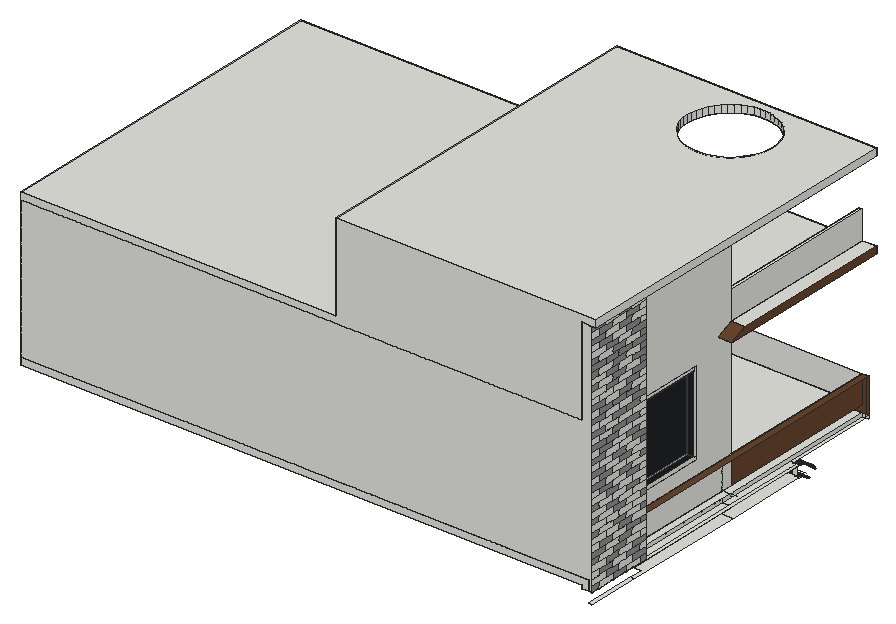
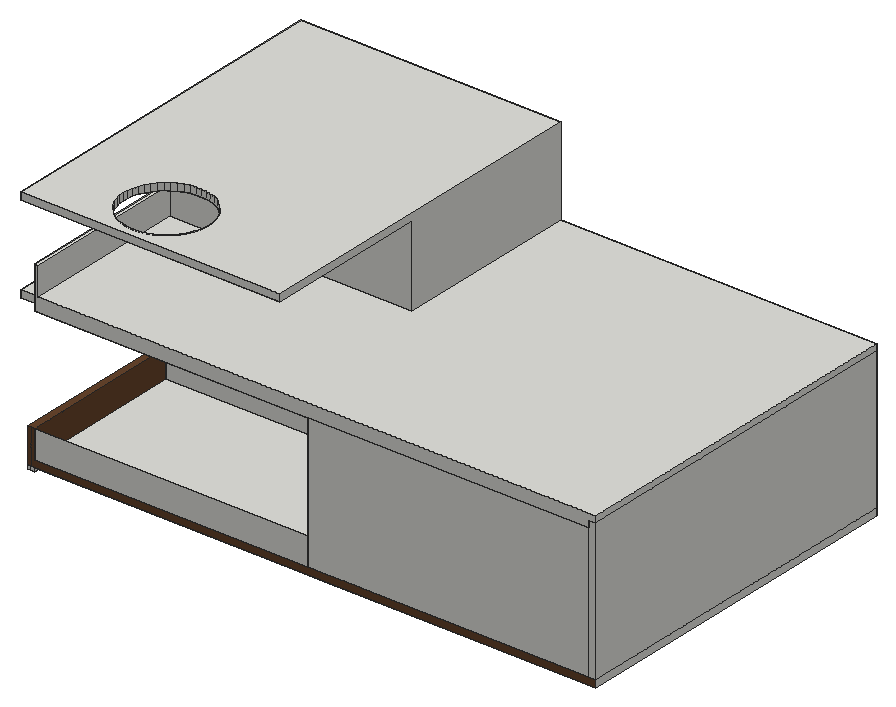
# SketchUp Ruby script. Lengths in inches.
U = 1.inch
M = Sketchup.active_model
def pt(a) = Geom::Point3d.new(a.map { |v| v * U })
def face(e, loops, mat)
  f = e.add_face(loops[0].map { |a| pt(a) })
  loops[1..].each { |l| e.add_face(l.map { |a| pt(a) }).erase! }
  f.material = f.back_material = mat if mat
  f
end
# faces: each face lists its corners as indices into pts; further lists are holes
def faces(e, pts, list, mat = nil) = list.each { |f| face(e, (f[0].is_a?(Array) ? f : [f]).map { |l| l.map { |i| pts[i] } }, mat) }
# xy, xz, yz: faces in a plane at the given z, y or x. An outline is a flat list of corners, or four numbers for a rectangle; further outlines are holes
def ring(l) = l.size == 4 ? [[l[0], l[1]], [l[2], l[1]], [l[2], l[3]], [l[0], l[3]]] : l.each_slice(2).to_a
def flat(e, list, mat, &to3) = list.each { |f| face(e, (f[0].is_a?(Array) ? f : [f]).map { |l| ring(l).map { |u, v| to3.(u, v) } }, mat) }
def xy(e, z, list, mat = nil) = flat(e, list, mat) { |x, y| [x, y, z] }
def xz(e, y, list, mat = nil) = flat(e, list, mat) { |x, z| [x, y, z] }
def yz(e, x, list, mat = nil) = flat(e, list, mat) { |y, z| [x, y, z] }
def lines(e, pts, list) = list.each { |a, b| e.add_line(pt(pts[a]), pt(pts[b])) }
# prism: a flat outline (further loops are holes) pulled along v
def prism(e, loops, v, mat = nil)
  f = face(e, loops, mat); d = Geom::Vector3d.new(v.map { |x| x * U })
  f.pushpull(f.normal.samedirection?(d) ? d.length : -d.length)
end
def box(e, o, s, mat = nil) = prism(e, [[o, [o[0] + s[0], o[1], o[2]], [o[0] + s[0], o[1] + s[1], o[2]], [o[0], o[1] + s[1], o[2]]]], [0, 0, s[2]], mat)
def at(x, y, z, deg = 0) = Geom::Transformation.translation(pt([x, y, z])) * Geom::Transformation.rotation(ORIGIN, Z_AXIS, deg.degrees)
def axes(o, x, y, z) = Geom::Transformation.new([*x, 0, *y, 0, *z, 0, *pt(o).to_a, 1])
def part(name) = M.definitions.add(name)
# library, detail: a bought-in or finely detailed component or shape, given as its bounding box
def library(name, o, s) = part(name).tap { |d| box(d.entities, o, s) }
def detail(e, o, s) = box(e.add_group.entities, o, s)
def put(e, d, t, mat = nil) = e.add_instance(d, t).tap { |i| i.material = mat if mat }
def group(e, t, mat = nil) = e.add_group.tap { |g| g.transformation = t; g.material = mat if mat }.entities
root = M.entities
M.materials.add("Glass_Basic_01").color = [130, 139, 150]
M.materials["Glass_Basic_01"].alpha = 0.25
M.materials.add("M04_Stone_Frost").color = [142, 142, 142]
M.materials.add("M09_Shadow_Night").color = [0, 0, 0]
M.materials.add("Wood_Veneer_15_1K").color = [103, 69, 45]
c1 = library("porta+4",[0.2,-5.42,1.33],[46.55,4.72,83.21])
c2 = library("mesh-166",[-1553.69,-2604.3125,-42.18],[1702.88,1401.6,88.28])
c3 = part("Group17")
put(c3.entities,c2,at(294.66,859.51,3.5))
prism(root,[[[276,153,504],[276,6,504],[474,6,504],[474,45,504],[474,153,504]]],[0,0,66])
xy(root,357,[[474,63,480,120]],"M09_Shadow_Night")
xy(root,360,[[486,0,489,45],[486,45,486,57,480,57,480,150,489,150,489,45],[480,150,480,159,477,159,477,222.15,489,222.15,489,150],[480,238.07,486,238.08]])
xy(root,368.99,[[486,0,489,45]])
xy(root,369,[[480,0,486,45],[486,0,489,45],[480,45,486,150],[486,45,489,57],[486,57,489,222.39],
  [480,150,486,222.39],[477,159,480,222.39],[480,222.39,483,300]])
xy(root,372,[[0,0,474,6],[474,0,480,159],[0,6,6,300],[6,6,6,294,240,294,240,153,474,153,474,6],[240,153,474,153,474,159,246,159,246,300,240,300],
  [246,159,480,300],[6,294,240,300]])
xy(root,378,[[[0,0,486,0,486,45,480,45,480,159,246,159,246,300,6,300,6,294,240,294,240,159,6,159,6,300,0,300],[6,6,474,153]],[6,6,474,153],[6,159,240,294],[246,159,480,300]])
xy(root,381,[[273,153,315,159]])
xy(root,402,[[480,45,486,57]])
xy(root,402,[[480,57,486,300]],"Wood_Veneer_15_1K")
xy(root,417,[[240,198,246,240]])
xy(root,417,[[474,63,480,120]],"M09_Shadow_Night")
xy(root,459,[[273,153,315,159],[240,198,246,240]])
xy(root,483,[[474,63,480,120]],"M09_Shadow_Night")
xy(root,492,[[6,6,474,153],[6,153,240,159],[240,159,240,294,6,294,6,300,246,300,246,159],[6,159,240,294],[246,159,474,300],
  [474,159,480,300]])
xy(root,498,[[0,0,6,300],[6,0,480,6],[480,145.31,492,159],[240,153,474,159],[480,159,492,300]])
xy(root,504,[[0,0,270,0,270,159,477,159,477,300,0,300],[480,159,492,300]])
xy(root,528,[[477,159,480,300]])
xy(root,573,[[480,0,489,6],[489,0,492,45],[480,6,489,57],[489,45,489,57,480,57,480,159,492,159,492,45],[[270,159,492,300],[400.57,221.16,405.09,221.33,409.55,222.08,413.88,223.375,418.01,225.2,421.89,227.53,425.4375,230.33,428.61,233.56,431.35,237.15,433.62,241.06,435.38,245.22,436.61,249.57,437.28,254.05,437.39,258.57,436.92,263.0625,435.9,267.47,434.34,271.71,432.25,275.72,429.68,279.4375,426.66,282.81,423.25,285.77,419.49,288.28,415.45,290.3,411.18,291.8,406.76,292.75,402.26,293.14,397.74,292.96,393.28,292.22,388.95,290.92,384.8125,289.09,380.94,286.76,377.39,283.96,374.22,280.74,371.48,277.14,369.21,273.23,367.45,269.07,366.22,264.72,365.55,260.25,365.44,255.73,365.9,251.23,366.92,246.83,368.49,242.59,370.57,238.57,373.15,234.86,376.16,231.49,379.58,228.53,383.34,226.01,387.38,223.99,391.65,222.5,396.07,221.55]]])
xy(root,579,[[[270,0,492,300],[400.57,221.16,396.07,221.55,391.65,222.5,387.38,223.99,383.34,226.01,379.58,228.53,376.16,231.49,373.15,234.86,370.57,238.57,368.49,242.59,366.92,246.83,365.9,251.23,365.44,255.73,365.55,260.25,366.22,264.72,367.45,269.07,369.21,273.23,371.48,277.14,374.22,280.74,377.39,283.96,380.94,286.76,384.8125,289.09,388.95,290.92,393.28,292.22,397.74,292.96,402.26,293.14,406.76,292.75,411.18,291.8,415.45,290.3,419.49,288.28,423.25,285.77,426.66,282.81,429.68,279.4375,432.25,275.72,434.34,271.71,435.9,267.47,436.92,263.0625,437.39,258.57,437.28,254.05,436.61,249.57,435.38,245.22,433.62,241.06,431.35,237.15,428.61,233.56,425.4375,230.33,421.89,227.53,418.01,225.2,413.88,223.375,409.55,222.08,405.09,221.33]]])
xz(root,0,[[486,368.99,489,369],[480,369,486,369,486,378,0,378,0,372,480,372],[486,369,489,369,489,573,480,573,480,498,0,498,0,378,486,378],[0,498,480,498,480,573,492,573,492,579,270,579,270,504,0,504]])
xz(root,6,[[6,378,474,492],[6,492,474,498]])
xz(root,45,[[486,368.99,489,369],[480,378,486,402]])
xz(root,57,[[486,369,486,402,480,402,480,573,489,573,489,369]])
xz(root,63,[[474,417,480,483]],"M09_Shadow_Night")
xz(root,120,[[474,417,480,483]],"M09_Shadow_Night")
xz(root,153,[[[6,378,474,492],[273,381,315,459]],[240,492,474,498]])
xz(root,159,[[6,378,240,492],[246,378,246,492,480,492,480,378,318,378,318,462,270,462,270,378],[[270,378,318,462],[273,381,315,459]],[240,492,246,498],[246,492,474,498],
  [474,492,480,498],[270,504,270,573,480,573,480,528,477,528,477,504]])
xz(root,198,[[240,417,246,459]])
xz(root,222.39,[[483,359.99,486,368.92],[477,368.92,483,368.97],[483,368.92,486,368.97],[486,368.92,489,368.97],[477,368.97,483,369],
  [483,368.97,486,369],[486,368.97,489,369]])
xz(root,240,[[240,417,246,459]])
xz(root,294,[[6,378,240,402],[6,402,240,492]])
xz(root,300,[[480,369,483,372],[483,369,486,372],[0,378,6,498],[6,378,246,492],[246,378,480,402],
  [6,492,6,498,0,498,0,504,477,504,477,528,480,528,480,492],[480,498,492,504],[270,573,492,579]])
xz(root,300,[[0,372,0,378,480,378,480,402,483,402,483,372],[483,372,486,402]],"Wood_Veneer_15_1K")
yz(root,0,[[0,372,300,378],[0,378,300,498],[0,498,300,504]])
yz(root,6,[[6,378,153,492],[153,378,159,492],[159,378,294,492],[6,492,300,498]])
yz(root,240,[[[159,378,294,492],[198,417,240,459]],[153,492,159,498]])
yz(root,246,[[[159,378,300,492],[195,414,243,462]],[[195,414,243,462],[198,417,240,459]]])
yz(root,270,[[0,504,0,579,300,579,300,573,159,573,159,504]])
yz(root,273,[[153,381,159,459]])
yz(root,315,[[153,381,159,459]])
yz(root,474,[[[6,378,153,492],[63,417,120,483]],[6,492,153,498]])
yz(root,474,[[63,417,120,483]],"M09_Shadow_Night")
yz(root,477,[[159,504,300,528]])
yz(root,480,[[0,369,45,372],[45,369,150,372],[150,369,159,372],[159,369,300,372],[45,378,150,402],
  [150,378,159,402],[[57,402,159,402,159,498,145.31,498,159,504,159,573,57,573],[63,417,120,483]],[159,492,300,498],[0,498,6,573],[6,498,57,573],
  [145.31,498,300,498,300,504,159,504],[159,504,300,528]])
yz(root,480,[[63,417,120,483]],"Glass_Basic_01")
yz(root,480,[[159,378,300,402]],"Wood_Veneer_15_1K")
yz(root,486,[[238.14,359.9,238.07,360,238.08,360],[0,368.99,45,369],[45,369,57,402]])
yz(root,486,[[0,369,45,378]],"Wood_Veneer_15_1K")
yz(root,489,[[238.91,358.58,238.7,358.97,238.48,359.35,238.25,359.72,238.14,359.9],[220.77,360,222.15,360,222.08,360,221.56,360.02,221.29,360.02],[222.39,368.97,222.39,369,214.74,369],[0,368.99,6.98,369],[6.98,368.99,21.65,369],
  [21.65,368.99,36.33,369],[36.33,368.99,45,369],[45,368.99,51,369],[51,368.99,57,369],[6.98,369,21.65,374.09],
  [36.33,369,51,374.09],[0,374.09,14.25,379.19],[28.5,374.09,42.75,379.19],[0,379.19,6.98,384.29],[21.65,379.19,36.33,384.29],
  [51,379.19,57,384.29],[0,384.29,14.25,389.39],[28.5,384.29,42.75,389.39],[6.98,389.39,21.65,394.49],[36.33,389.39,51,394.49],
  [51,389.39,57,394.49],[14.25,394.49,28.5,399.59],[42.75,394.49,57,399.59],[0,399.59,6.98,404.69],[21.65,399.59,36.33,404.69],
  [0,404.69,14.25,409.79],[14.25,404.69,28.5,409.79],[42.75,404.69,57,409.79],[6.98,409.79,21.65,414.89],[36.33,409.79,51,414.89],
  [0,414.89,14.25,419.99],[14.25,414.89,28.5,419.99],[28.5,414.89,42.75,419.99],[42.75,414.89,57,419.99],[6.98,419.99,21.65,425.09],
  [36.33,419.99,51,425.09],[0,425.09,14.25,430.19],[28.5,425.09,42.75,430.19],[42.75,425.09,57,430.19],[6.98,430.19,21.65,435.29],
  [21.65,430.19,36.33,435.29],[51,430.19,57,435.29],[0,435.29,14.25,440.39],[28.5,435.29,42.75,440.39],[42.75,435.29,57,440.39],
  [0,440.39,6.98,445.49],[21.65,440.39,36.33,445.49],[51,440.39,57,445.49],[14.25,445.49,28.5,450.59],[42.75,445.49,57,450.59],
  [0,450.59,6.98,455.69],[21.65,450.59,36.33,455.69],[36.33,450.59,51,455.69],[14.25,455.69,28.5,460.79],[42.75,455.69,57,460.79],
  [0,460.79,6.98,465.9],[6.98,460.79,21.65,465.9],[36.33,460.79,51,465.9],[14.25,465.9,28.5,471],[28.5,465.9,42.75,471],
  [0,471,6.98,476.1],[21.65,471,36.33,476.1],[51,471,57,476.1],[28.5,476.1,42.75,481.2],[42.75,476.1,57,481.2],
  [0,481.2,6.98,486.3],[6.98,481.2,21.65,486.3],[51,481.2,57,486.3],[14.25,486.3,28.5,491.4],[28.5,486.3,42.75,491.4],
  [42.75,486.3,57,491.4],[0,491.4,6.98,496.5],[6.98,491.4,21.65,496.5],[51,491.4,57,496.5],[14.25,496.5,28.5,501.6],
  [28.5,496.5,42.75,501.6],[0,501.6,6.98,506.7],[51,501.6,57,506.7],[14.25,506.7,28.5,511.8],[42.75,506.7,57,511.8],
  [0,511.8,6.98,516.9],[6.98,511.8,21.65,516.9],[21.65,511.8,36.33,516.9],[51,511.8,57,516.9],[0,516.9,14.25,522],
  [28.5,516.9,42.75,522],[6.98,522,21.65,527.1],[36.33,522,51,527.1],[0,527.1,14.25,532.2],[28.5,527.1,42.75,532.2],
  [6.98,532.2,21.65,537.3],[36.33,532.2,51,537.3],[6.98,542.4,21.65,547.5],[36.33,542.4,51,547.5],[0,547.5,14.25,552.6],
  [28.5,547.5,42.75,552.6],[0,552.6,6.98,557.7],[21.65,552.6,36.33,557.7],[51,552.6,57,557.7],[14.25,557.7,28.5,562.8],
  [42.75,557.7,57,562.8],[0,562.8,6.98,567.9],[21.65,562.8,36.33,567.9],[51,562.8,57,567.9],[14.25,567.9,28.5,573],
  [42.75,567.9,57,573]])
yz(root,489,[[0,369,6.98,374.09],[21.65,369,36.33,374.09],[51,369,57,374.09],[14.25,374.09,28.5,379.19],[42.75,374.09,57,379.19],
  [6.98,379.19,21.65,384.29],[36.33,379.19,51,384.29],[14.25,384.29,28.5,389.39],[42.75,384.29,57,389.39],[0,389.39,6.98,394.49],
  [21.65,389.39,36.33,394.49],[0,394.49,14.25,399.59],[28.5,394.49,42.75,399.59],[6.98,399.59,21.65,404.69],[36.33,399.59,51,404.69],
  [51,399.59,57,404.69],[28.5,404.69,42.75,409.79],[0,409.79,6.98,414.89],[21.65,409.79,36.33,414.89],[51,409.79,57,414.89],
  [0,419.99,6.98,425.09],[21.65,419.99,36.33,425.09],[51,419.99,57,425.09],[14.25,425.09,28.5,430.19],[0,430.19,6.98,435.29],
  [36.33,430.19,51,435.29],[14.25,435.29,28.5,440.39],[6.98,440.39,21.65,445.49],[36.33,440.39,51,445.49],[0,445.49,14.25,450.59],
  [28.5,445.49,42.75,450.59],[6.98,450.59,21.65,455.69],[51,450.59,57,455.69],[0,455.69,14.25,460.79],[28.5,455.69,42.75,460.79],
  [21.65,460.79,36.33,465.9],[51,460.79,57,465.9],[0,465.9,14.25,471],[42.75,465.9,57,471],[6.98,471,21.65,476.1],
  [36.33,471,51,476.1],[0,476.1,14.25,481.2],[14.25,476.1,28.5,481.2],[21.65,481.2,36.33,486.3],[36.33,481.2,51,486.3],
  [0,486.3,14.25,491.4],[21.65,491.4,36.33,496.5],[36.33,491.4,51,496.5],[0,496.5,14.25,501.6],[42.75,496.5,57,501.6],
  [6.98,501.6,21.65,506.7],[21.65,501.6,36.33,506.7],[36.33,501.6,51,506.7],[0,506.7,14.25,511.8],[28.5,506.7,42.75,511.8],
  [36.33,511.8,51,516.9],[14.25,516.9,28.5,522],[42.75,516.9,57,522],[0,522,6.98,527.1],[21.65,522,36.33,527.1],
  [51,522,57,527.1],[14.25,527.1,28.5,532.2],[42.75,527.1,57,532.2],[0,532.2,6.98,537.3],[21.65,532.2,36.33,537.3],
  [51,532.2,57,537.3],[0,537.3,14.25,542.4],[14.25,537.3,28.5,542.4],[28.5,537.3,42.75,542.4],[42.75,537.3,57,542.4],
  [0,542.4,6.98,547.5],[21.65,542.4,36.33,547.5],[51,542.4,57,547.5],[14.25,547.5,28.5,552.6],[42.75,547.5,57,552.6],
  [6.98,552.6,21.65,557.7],[36.33,552.6,51,557.7],[0,557.7,14.25,562.8],[28.5,557.7,42.75,562.8],[6.98,562.8,21.65,567.9],
  [36.33,562.8,51,567.9],[0,567.9,14.25,573],[28.5,567.9,42.75,573]],"M04_Stone_Frost")
yz(root,492,[[0,573,300,579]])
yz(root,492,[[145.31,498,300,498,300,504,159,504]],"Wood_Veneer_15_1K")
p = [[486,232.23,354.64],[489,232.23,354.64],[489,232.07,354.85],[477,232.07,354.85],[477,232.23,354.64],[483,232.23,354.64],
  [486,232.09,354.83],[483,232.09,354.83],[486,231.95,355.01],[483,231.95,355.01],[489,231.91,355.06],[477,231.91,355.06],
  [486,231.8,355.18],[483,231.8,355.18],[489,231.74,355.26],[477,231.74,355.26],[486,231.65,355.36],[483,231.65,355.36],
  [489,231.57,355.46],[477,231.57,355.46],[486,231.49,355.53],[483,231.49,355.53],[486,231.34,355.7],[483,231.34,355.7],
  [489,231.39,355.66],[477,231.39,355.66],[489,231.21,355.85],[477,231.21,355.85],[486,231.18,355.87],[483,231.18,355.87],
  [489,231.03,356.04],[477,231.03,356.04],[486,231.01,356.03],[483,231.01,356.03],[489,230.84,356.22],[477,230.84,356.22],
  [486,230.85,356.2],[483,230.85,356.2],[489,230.65,356.4],[477,230.65,356.4],[486,230.68,356.36],[483,230.68,356.36],
  [489,230.46,356.58],[477,230.46,356.58],[486,230.51,356.51],[483,230.51,356.51],[486,230.33,356.67],[483,230.33,356.67],
  [489,230.26,356.76],[477,230.26,356.76],[486,230.16,356.82],[483,230.16,356.82],[486,229.98,356.96],[483,229.98,356.96],
  [489,230.06,356.92],[477,230.06,356.92],[489,229.85,357.09],[477,229.85,357.09],[486,229.8,357.11],[483,229.8,357.11],
  [489,229.64,357.25],[477,229.64,357.25],[486,229.62,357.25],[483,229.62,357.25],[486,229.43,357.39],[483,229.43,357.39],
  [489,229.43,357.41],[477,229.43,357.41],[489,229.22,357.5625],[477,229.22,357.5625],[486,229.24,357.52],[483,229.24,357.52],
  [486,229.05,357.65],[483,229.05,357.65],[489,229,357.71],[477,229,357.71],[489,228.78,357.86],[477,228.78,357.86],
  [486,228.86,357.78],[483,228.86,357.78],[486,228.66,357.91],[483,228.66,357.91],[486,228.47,358.03],[483,228.47,358.03],
  [489,228.56,358],[477,228.56,358],[489,228.33,358.14],[477,228.33,358.14],[486,228.27,358.15],[483,228.27,358.15],
  [489,228.11,358.27],[477,228.11,358.27],[486,228.07,358.26],[483,228.07,358.26],[489,227.875,358.4],[477,227.875,358.4],
  [486,227.86,358.375],[483,227.86,358.375],[489,227.64,358.52],[477,227.64,358.52],[486,227.66,358.48],[483,227.66,358.48],
  [489,227.41,358.64],[477,227.41,358.64],[486,227.45,358.59],[483,227.45,358.59],[489,227.17,358.75],[477,227.17,358.75],
  [486,227.24,358.69],[483,227.24,358.69],[486,227.03,358.79],[483,227.03,358.79],[486,226.82,358.88],[483,226.82,358.88],
  [489,226.93,358.86],[477,226.93,358.86],[486,226.61,358.97],[483,226.61,358.97],[489,226.6875,358.96],[477,226.6875,358.96],
  [489,226.44,359.06],[477,226.44,359.06],[486,226.4,359.0625],[483,226.4,359.0625],[486,226.18,359.14],[486,225.96,359.22],
  [483,225.96,359.22],[483,226.18,359.14],[489,226.2,359.16],[477,226.2,359.16],[477,225.95,359.25],[489,225.95,359.25],
  [489,225.7,359.33],[477,225.7,359.33],[486,225.74,359.3],[483,225.74,359.3],[489,225.45,359.42],[477,225.45,359.42],
  [486,225.52,359.37],[483,225.52,359.37],[486,225.3,359.44],[486,225.08,359.51],[483,225.08,359.51],[483,225.3,359.44],
  [489,225.2,359.49],[477,225.2,359.49],[489,224.94,359.5625],[477,224.94,359.5625],[486,224.86,359.57],[483,224.86,359.57],
  [477,224.6875,359.625],[489,224.6875,359.625],[489,224.43,359.6875],[477,224.43,359.6875],[486,224.63,359.625],[486,224.41,359.68],
  [483,224.41,359.68],[483,224.63,359.625],[477,224.17,359.74],[489,224.17,359.74],[489,223.92,359.79],[477,223.92,359.79],
  [486,224.18,359.73],[486,223.95,359.77],[483,223.95,359.77],[483,224.18,359.73],[477,223.66,359.84],[489,223.66,359.84],
  [489,223.4,359.88],[477,223.4,359.88],[486,223.73,359.82],[486,223.5,359.86],[483,223.5,359.86],[483,223.73,359.82],
  [477,222.87,359.94],[489,222.87,359.94],[489,222.61,359.97],[477,222.61,359.97],[486,222.81,359.95],[486,222.58,359.97],
  [483,222.58,359.97],[483,222.81,359.95],[486,223.04,359.92],[483,223.04,359.92],[477,223.13,359.91],[489,223.13,359.91],
  [486,223.27,359.89],[483,223.27,359.89],[477,238.01,360.09],[489,238.01,360.09],[489,238.14,359.9],[486,238.14,359.9],
  [486,238.07,360],[480,238.07,360],[477,238.07,360],[477,238.14,359.9],[477,222.35,359.99],[486,222.35,359.99],
  [486,222.15,360],[477,222.15,360],[489,222.15,360],[489,222.35,359.99],[486,222.39,359.99],[483,222.39,359.99],
  [477,237.76,360.46],[489,237.76,360.46],[477,237.51,360.82],[489,237.51,360.82],[477,237.25,361.17],[489,237.25,361.17],
  [477,236.98,361.52],[489,236.98,361.52],[477,236.7,361.86],[489,236.7,361.86],[477,236.41,362.19],[489,236.41,362.19],
  [477,236.12,362.52],[489,236.12,362.52],[477,235.82,362.85],[489,235.82,362.85],[477,235.51,363.16],[489,235.51,363.16],
  [477,235.2,363.47],[489,235.2,363.47],[477,234.875,363.77],[489,234.875,363.77],[477,234.55,364.0625],[489,234.55,364.0625],
  [477,234.21,364.35],[489,234.21,364.35],[477,233.875,364.63],[489,233.875,364.63],[477,233.53,364.9],[489,233.53,364.9],
  [477,233.17,365.16],[489,233.17,365.16],[477,232.81,365.42],[489,232.81,365.42],[477,232.45,365.67],[489,232.45,365.67],
  [477,232.08,365.9],[489,232.08,365.9],[477,231.71,366.14],[489,231.71,366.14],[477,231.33,366.36],[489,231.33,366.36],
  [477,230.94,366.57],[489,230.94,366.57],[477,230.55,366.78],[489,230.55,366.78],[477,230.16,366.97],[489,230.16,366.97],
  [477,229.76,367.16],[489,229.76,367.16],[477,229.36,367.34],[489,229.36,367.34],[477,228.95,367.51],[489,228.95,367.51],
  [477,229.08,367.45],[477,228.54,367.67],[489,228.54,367.67],[477,228.125,367.82],[489,228.125,367.82],[477,227.71,367.96],
  [489,227.71,367.96],[477,227.29,368.09],[489,227.29,368.09],[477,226.87,368.21],[489,226.87,368.21],[477,226.44,368.33],
  [489,226.44,368.33],[477,226.01,368.43],[489,226.01,368.43],[477,225.58,368.53],[489,225.58,368.53],[477,225.15,368.61],
  [489,225.15,368.61],[477,224.72,368.69],[489,224.72,368.69],[477,224.28,368.75],[489,224.28,368.75],[477,223.41,368.85],
  [489,223.41,368.85],[489,223.84,368.81],[477,223.84,368.81],[486,222.39,368.92],[489,222.39,368.92],[489,222.53,368.91],
  [477,222.53,368.91],[477,222.39,368.92],[483,222.39,368.92],[489,222.97,368.89],[477,222.97,368.89],[480,159,504],
  [480,145.31,498],[492,145.31,498],[492,159,504],[396.07,221.55,579],[400.57,221.16,579],[400.57,221.16,573],
  [396.07,221.55,573],[405.09,221.33,579],[405.09,221.33,573],[409.55,222.08,579],[409.55,222.08,573],[391.65,222.5,579],
  [391.65,222.5,573],[413.88,223.375,579],[413.88,223.375,573],[387.38,223.99,579],[387.38,223.99,573],[418.01,225.2,579],
  [418.01,225.2,573],[383.34,226.01,579],[383.34,226.01,573],[421.89,227.53,579],[421.89,227.53,573],[379.58,228.53,579],
  [379.58,228.53,573],[425.4375,230.33,579],[425.4375,230.33,573],[376.16,231.49,579],[376.16,231.49,573],[428.61,233.56,579],
  [428.61,233.56,573],[373.15,234.86,579],[373.15,234.86,573],[431.35,237.15,579],[431.35,237.15,573],[370.57,238.57,579],
  [370.57,238.57,573],[433.62,241.06,579],[433.62,241.06,573],[368.49,242.59,579],[368.49,242.59,573],[435.38,245.22,579],
  [435.38,245.22,573],[366.92,246.83,579],[366.92,246.83,573],[436.61,249.57,579],[436.61,249.57,573],[365.9,251.23,579],
  [365.9,251.23,573],[437.28,254.05,579],[437.28,254.05,573],[365.44,255.73,579],[365.44,255.73,573],[437.39,258.57,579],
  [437.39,258.57,573],[365.55,260.25,579],[365.55,260.25,573],[436.92,263.0625,579],[436.92,263.0625,573],[366.22,264.72,579],
  [366.22,264.72,573],[435.9,267.47,579],[435.9,267.47,573],[367.45,269.07,579],[367.45,269.07,573],[434.34,271.71,579],
  [434.34,271.71,573],[369.21,273.23,579],[369.21,273.23,573],[432.25,275.72,579],[432.25,275.72,573],[371.48,277.14,579],
  [371.48,277.14,573],[429.68,279.4375,579],[429.68,279.4375,573],[374.22,280.74,579],[374.22,280.74,573],[426.66,282.81,579],
  [426.66,282.81,573],[377.39,283.96,579],[377.39,283.96,573],[423.25,285.77,579],[423.25,285.77,573],[380.94,286.76,579],
  [380.94,286.76,573],[419.49,288.28,579],[419.49,288.28,573],[384.8125,289.09,579],[384.8125,289.09,573],[415.45,290.3,579],
  [415.45,290.3,573],[388.95,290.92,579],[388.95,290.92,573],[411.18,291.8,579],[411.18,291.8,573],[393.28,292.22,579],
  [393.28,292.22,573],[406.76,292.75,579],[406.76,292.75,573],[397.74,292.96,579],[397.74,292.96,573],[402.26,293.14,579],
  [402.26,293.14,573],[246,159,498],[240,159,498],[480,45,372],[486,45,372],[480,159,372],
  [486,159,372],[489,208.82,369],[489,208.82,369.03],[489,229.08,360],[477,229.08,360],[480,229.08,367.45],
  [480,45,378],[480,45,377.91],[480,123,414],[480,123,417],[480,60.02,483],[480,60.02,486],
  [480,120,486],[480,63,483],[480,60.02,417.125],[480,60.02,417],[480,60.02,414],[480,63,417],
  [480,123,486],[480,120,483],[480,120,417]]
faces(root,p,[[0,1,2,3,4,5],[0,6,7,5],[6,8,9,7],[3,2,10,11],[8,12,13,9],[11,10,14,15],[12,16,17,13],[15,14,18,19],
  [16,20,21,17],[20,22,23,21],[19,18,24,25],[25,24,26,27],[22,28,29,23],[27,26,30,31],[28,32,33,29],[31,30,34,35],
  [32,36,37,33],[35,34,38,39],[36,40,41,37],[39,38,42,43],[40,44,45,41],[44,46,47,45],[43,42,48,49],[46,50,51,47],
  [50,52,53,51],[49,48,54,55],[55,54,56,57],[52,58,59,53],[57,56,60,61],[58,62,63,59],[62,64,65,63],[61,60,66,67],
  [67,66,68,69],[64,70,71,65],[70,72,73,71],[69,68,74,75],[75,74,76,77],[72,78,79,73],[78,80,81,79],[80,82,83,81],
  [77,76,84,85],[85,84,86,87],[82,88,89,83],[87,86,90,91],[88,92,93,89],[91,90,94,95],[92,96,97,93],[95,94,98,99],
  [96,100,101,97],[99,98,102,103],[100,104,105,101],[103,102,106,107],[104,108,109,105],[108,110,111,109],[110,112,113,111],[107,106,114,115],
  [112,116,117,113],[115,114,118,119],[119,118,120,121],[116,122,123,117],[124,125,126,127],[121,120,128,129],[122,124,127,123],[130,131,132,133],
  [125,134,135,126],[129,128,131,130],[133,132,136,137],[134,138,139,135],[140,141,142,143],[137,136,144,145],[138,140,143,139],[145,144,146,147],
  [141,148,149,142],[150,151,152,153],[154,155,156,157],[148,154,157,149],[147,146,151,150],[158,159,160,161],[162,163,164,165],[153,152,159,158],
  [155,162,165,156],[166,167,168,169],[170,171,172,173],[161,160,167,166],[163,170,173,164],[174,175,176,177],[178,179,180,181],[182,178,181,183],
  [184,185,175,174],[186,182,183,187],[169,168,185,184],[171,186,187,172],[188,189,190,191,192,193,194],[192,191,195,194,193],[196,197,198,199],[200,198,197,201],
  [177,176,201,197,196],[179,202,203,180],[204,205,189,188],[206,207,205,204],[208,209,207,206],[210,211,209,208],[212,213,211,210],[214,215,213,212],
  [216,217,215,214],[218,219,217,216],[220,221,219,218],[222,223,221,220],[224,225,223,222],[226,227,225,224],[228,229,227,226],[230,231,229,228],
  [232,233,231,230],[234,235,233,232],[236,237,235,234],[238,239,237,236],[240,241,239,238],[242,243,241,240],[244,245,243,242],[246,247,245,244],
  [248,249,247,246],[250,251,249,248],[252,253,251,250],[254,255,253,252],[256,257,255,254,258],[259,260,257,256],[261,262,260,259],[263,264,262,261],
  [265,266,264,263],[267,268,266,265],[269,270,268,267],[271,272,270,269],[273,274,272,271],[275,276,274,273],[277,278,276,275],[279,280,278,277],
  [281,282,283,284],[284,283,280,279],[285,286,287,288,289,290],[288,287,291,292],[292,291,282,281],[297,298,299,300],[298,301,302,299],[301,303,304,302],
  [305,297,300,306],[303,307,308,304],[309,305,306,310],[307,311,312,308],[313,309,310,314],[311,315,316,312],[317,313,314,318],[315,319,320,316],
  [321,317,318,322],[319,323,324,320],[325,321,322,326],[323,327,328,324],[329,325,326,330],[327,331,332,328],[333,329,330,334],[331,335,336,332],
  [337,333,334,338],[335,339,340,336],[341,337,338,342],[339,343,344,340],[345,341,342,346],[343,347,348,344],[349,345,346,350],[347,351,352,348],
  [353,349,350,354],[351,355,356,352],[357,353,354,358],[355,359,360,356],[361,357,358,362],[359,363,364,360],[365,361,362,366],[363,367,368,364],
  [369,365,366,370],[367,371,372,368],[373,369,370,374],[371,375,376,372],[377,373,374,378],[375,379,380,376],[381,377,378,382],[379,383,384,380],
  [385,381,382,386],[383,387,388,384],[389,385,386,390],[387,391,392,388],[393,389,390,394],[391,395,396,392],[395,393,394,396]])
faces(root,p,[[293,294,295,296]],"Wood_Veneer_15_1K")
lines(root,p,[[397,398],[399,400],[401,402],[403,404],[405,406],[407,258],[202,197],[408,409],[410,411],[412,413],[414,413],[415,412],
  [412,416],[416,417],[418,417],[417,419],[410,418],[420,414],[414,421],[422,411],[411,420]])
put(root,c1,at(269.8,164.42,377.46))
put(root,c3,axes([247.52,230.5,474.45],[0,0.02817,0],[0,0,0.03465],[0.03937,0,0]))
